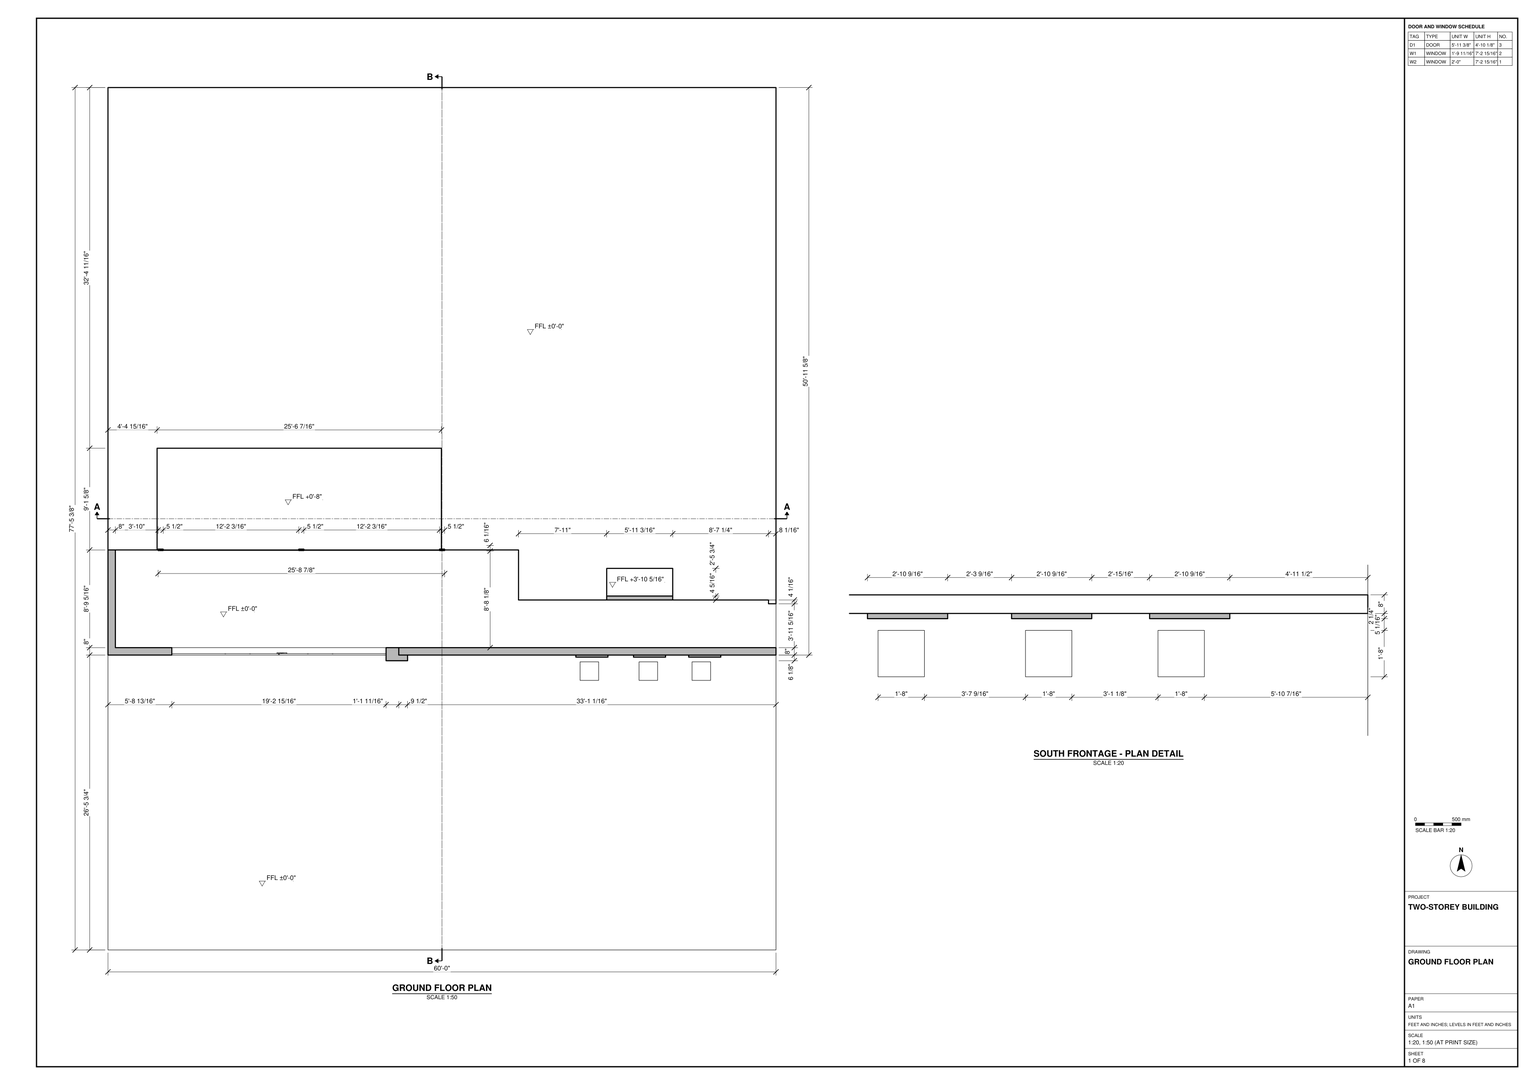
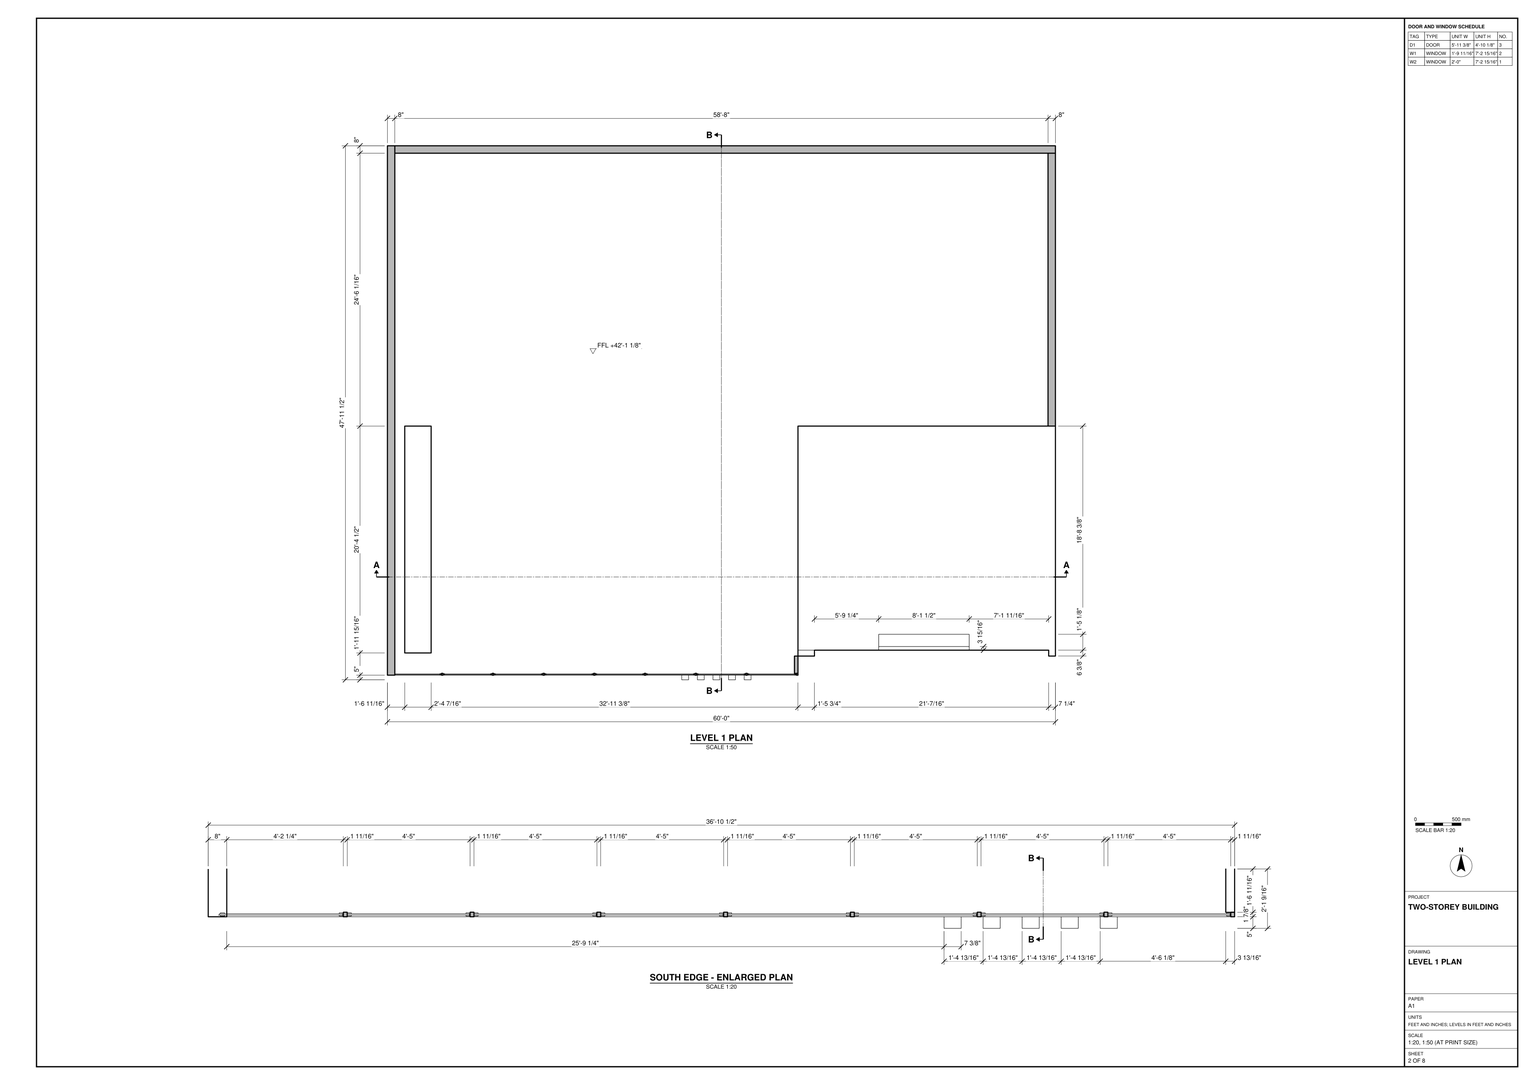
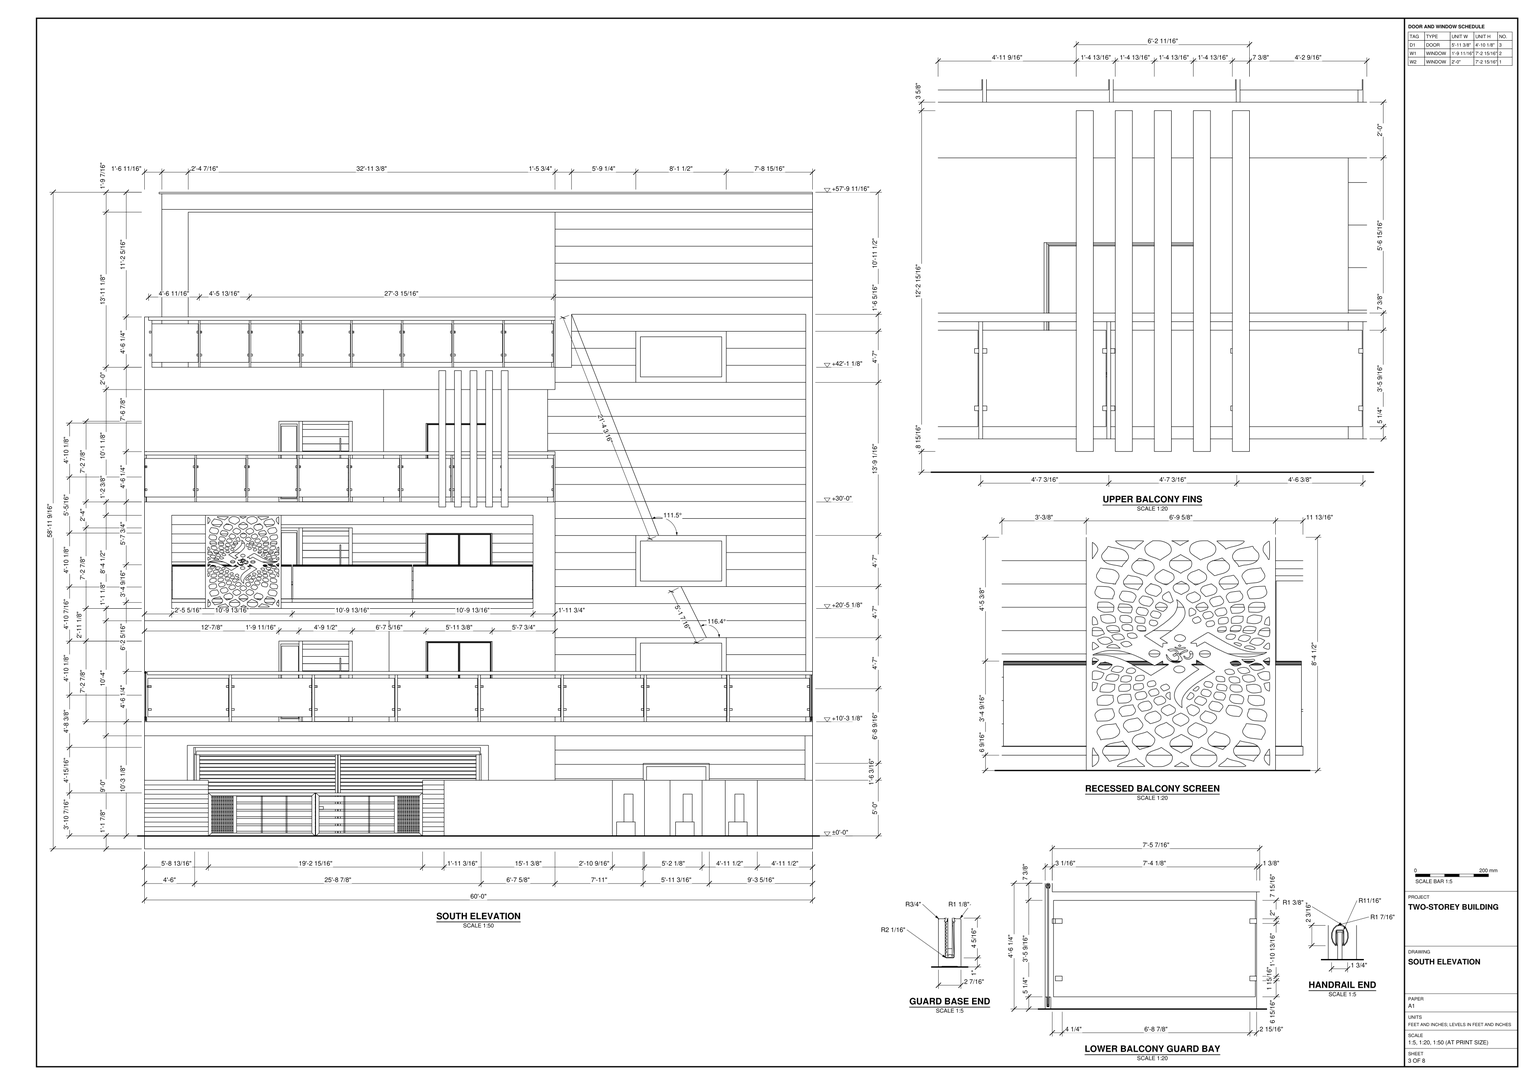
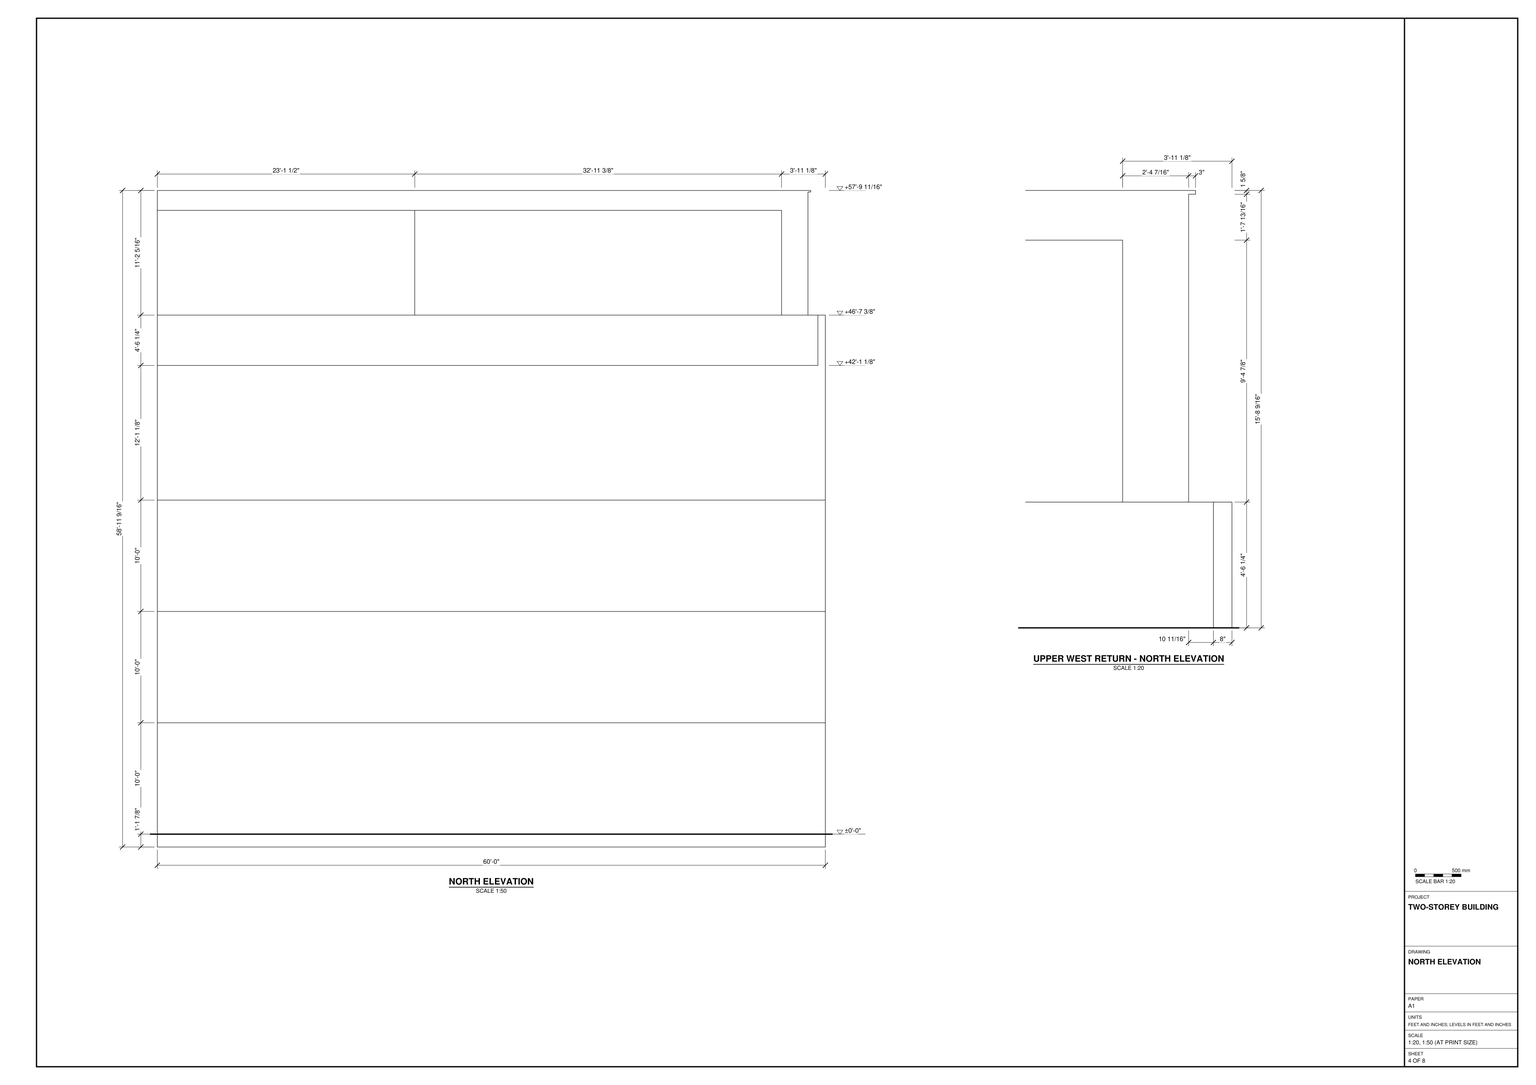
Build the two-storey building in SketchUp from task_files/diagram_01.pdf. Work in feet and inches. The complete model, including the ground area in front of the building, measures 60'-0" along X, 77'-5 3/8" along Y and 58'-11 9/16" in height. Set the ground floor at ±0'-0" and Level 1 at +42'-1 1/8". Use the south elevation to set the intermediate balcony heights rather than spacing the balconies evenly between the storey levels.

Follow the plans for the frontage setback, wall thicknesses, slab outlines and openings. Use the sections to establish slab and roof thicknesses. On the south face, model the wide ground-level gate, the full-width lower balcony and the shorter balconies above it. Include the framed doors and windows behind the guards. Reproduce the horizontal bands and window arrangement on the right-hand wall. Use the enlarged details to place the perforated screen in the recessed balcony and the vertical fins in front of the balcony above. Divide the glass guards into bays with posts and handrails as drawn.

Include stairs, built-in joinery and main furniture only where shown. Keep shell elements such as walls, slabs and roof, and each furniture or joinery piece, in separate groups or components. Use components for repeated parts such as guard bays. Decor and loose items may be any suitable library components. Save one SketchUp model as output_files/two_storey_building_with_stacked_south_facing_balconies.skp.

# SketchUp Ruby script. Lengths in inches.
U = 1.inch
M = Sketchup.active_model
def pt(a) = Geom::Point3d.new(a.map { |v| v * U })
def face(e, loops, mat)
  f = e.add_face(loops[0].map { |a| pt(a) })
  loops[1..].each { |l| e.add_face(l.map { |a| pt(a) }).erase! }
  f.material = f.back_material = mat if mat
  f
end
# faces: each face lists its corners as indices into pts; further lists are holes
def faces(e, pts, list, mat = nil) = list.each { |f| face(e, (f[0].is_a?(Array) ? f : [f]).map { |l| l.map { |i| pts[i] } }, mat) }
# xy, xz, yz: faces in a plane at the given z, y or x. An outline is a flat list of corners, or four numbers for a rectangle; further outlines are holes
def ring(l) = l.size == 4 ? [[l[0], l[1]], [l[2], l[1]], [l[2], l[3]], [l[0], l[3]]] : l.each_slice(2).to_a
def flat(e, list, mat, &to3) = list.each { |f| face(e, (f[0].is_a?(Array) ? f : [f]).map { |l| ring(l).map { |u, v| to3.(u, v) } }, mat) }
def xy(e, z, list, mat = nil) = flat(e, list, mat) { |x, y| [x, y, z] }
def xz(e, y, list, mat = nil) = flat(e, list, mat) { |x, z| [x, y, z] }
def yz(e, x, list, mat = nil) = flat(e, list, mat) { |y, z| [x, y, z] }
def lines(e, pts, list) = list.each { |a, b| e.add_line(pt(pts[a]), pt(pts[b])) }
# prism: a flat outline (further loops are holes) pulled along v
def prism(e, loops, v, mat = nil)
  f = face(e, loops, mat); d = Geom::Vector3d.new(v.map { |x| x * U })
  f.pushpull(f.normal.samedirection?(d) ? d.length : -d.length)
end
def box(e, o, s, mat = nil) = prism(e, [[o, [o[0] + s[0], o[1], o[2]], [o[0] + s[0], o[1] + s[1], o[2]], [o[0], o[1] + s[1], o[2]]]], [0, 0, s[2]], mat)
def at(x, y, z, deg = 0) = Geom::Transformation.translation(pt([x, y, z])) * Geom::Transformation.rotation(ORIGIN, Z_AXIS, deg.degrees)
def axes(o, x, y, z) = Geom::Transformation.new([*x, 0, *y, 0, *z, 0, *pt(o).to_a, 1])
def part(name) = M.definitions.add(name)
# library, detail: a bought-in or finely detailed component or shape, given as its bounding box
def library(name, o, s) = part(name).tap { |d| box(d.entities, o, s) }
def detail(e, o, s) = box(e.add_group.entities, o, s)
def put(e, d, t, mat = nil) = e.add_instance(d, t).tap { |i| i.material = mat if mat }
def group(e, t, mat = nil) = e.add_group.tap { |g| g.transformation = t; g.material = mat if mat }.entities
root = M.entities
M.materials.add("[0029_BlanchedAlmond]").color = [255, 235, 205]
M.materials.add("[0050_LemonChiffon]").color = [255, 250, 205]
M.materials.add("[0131_Silver]").color = [28, 28, 28]
M.materials.add("[0135_DarkGray]1").color = [81, 81, 81]
M.materials.add("[Color_000]").color = [255, 255, 255]
M.materials.add("[Granite Dark Gray]").color = [69, 68, 68]
M.materials.add("[Granite Light Gray]").color = [149, 148, 144]
M.materials.add("[Sandstone]").color = [118, 81, 52]
M.materials.add("[Slate Light Tile]").color = [53, 53, 53]
M.materials.add("[Translucent Glass Blue]").color = [100, 149, 237]
M.materials["[Translucent Glass Blue]"].alpha = 0.5
M.materials.add("[Translucent_Glass_Blue]").color = [255, 255, 255]
M.materials["[Translucent_Glass_Blue]"].alpha = 0
M.materials.add("[Wood Cherry Original]").color = [68, 39, 18]
M.materials.add("[Wood Cherry Original]1").color = [152, 86, 42]
M.materials.add("[Wood Floor Light]").color = [140, 99, 62]
c1 = part("Group\#11")
xy(c1.entities,0,[[0,0,0.39,2.125]],"[0131_Silver]")
xy(c1.entities,1.5,[[0,0,0.39,2.125]],"[0131_Silver]")
xz(c1.entities,0,[[0,0,0.39,1.5]],"[0131_Silver]")
xz(c1.entities,2.125,[[0,0,0.39,1.5]],"[0131_Silver]")
yz(c1.entities,0,[[0,0,2.125,1.5]],"[0131_Silver]")
yz(c1.entities,0.39,[[0,0,2.125,1.5]],"[0131_Silver]")
c2 = part("Glass railing panel")
xy(c2.entities,0,[[-0.59,0,0,63.98]])
xy(c2.entities,37.71,[[-0.59,0,0,63.98]])
xz(c2.entities,0,[[-0.59,0,0,37.71]])
xz(c2.entities,63.98,[[-0.59,0,0,37.71]])
yz(c2.entities,-0.59,[[0,0,63.98,37.71]])
yz(c2.entities,0,[[0,0,63.98,0,63.98,37.71,0,37.71,0,30.53,1.75,30.53,1.75,28.71,0,28.71],[-0.4,28.71,0,30.53],[0,28.71,1.75,30.53]])
p = [[0,63.98,30.53],[0.39,63.98,30.53]]
lines(c2.entities,p,[[0,1]])
put(c2.entities,c1,axes([0,62.22,28.71],[1,0,0],[0,1.01246,0],[0,0,1.2158]))
put(c2.entities,c1,axes([0,62.22,6.27],[1,0,0],[0,1.01246,0],[0,0,1.2158]))
put(c2.entities,c1,axes([0,0.6,28.71],[1,0,0],[0,1.01246,0],[0,0,1.2158]))
put(c2.entities,c1,axes([0,0.6,6.27],[1,0,0],[0,1.01246,0],[0,0,1.2158]))
put(c2.entities,c1,axes([-0.98,0.6,28.71],[1,0,0],[0,1.01246,0],[0,0,1.2158]))
put(c2.entities,c1,axes([-0.98,62.22,6.27],[1,0,0],[0,1.01246,0],[0,0,1.2158]))
put(c2.entities,c1,axes([-0.98,0.6,6.27],[1,0,0],[0,1.01246,0],[0,0,1.2158]))
put(c2.entities,c1,axes([-0.98,62.22,28.71],[1,0,0],[0,1.01246,0],[0,0,1.2158]))
c3 = part("Group\#1")
xz(c3.entities,0,[[0,0,1.97,38.58]])
xz(c3.entities,1.97,[[0,0,1.97,38.58]])
yz(c3.entities,0,[[0,0,1.97,37.71]])
yz(c3.entities,1.97,[[0,0,1.97,37.71]])
c4 = part("Glass railing run")
xy(c4.entities,37.71,[[2.51,0,3.15,0.39,3.15,0]])
xy(c4.entities,37.71,[[0,0,0.54,520.67],[2.51,0,2.51,63.58,3.15,0.39],[3.15,0.39,2.51,63.58,2.51,520.67,3.15,520.67]],"[0131_Silver]")
xy(c4.entities,38.58,[[0.54,496.0625,2.51,520.67]])
xy(c4.entities,38.58,[[0.54,0,2.51,496.0625]],"[0131_Silver]")
xy(c4.entities,40.46,[[0,0,3.15,520.67]],"[0131_Silver]")
xz(c4.entities,0,[[0,37.71,0.54,37.71,0.54,38.58,2.51,38.58,2.51,37.71,3.15,37.71,3.15,40.46,0,40.46]],"[0131_Silver]")
xz(c4.entities,520.67,[[0,37.71,0,40.46,3.15,40.46,3.15,37.71,2.51,37.71,2.51,38.58,0.54,38.58,0.54,37.71]])
yz(c4.entities,0,[[0,37.71,520.67,40.46]],"[0131_Silver]")
yz(c4.entities,0.54,[[496.0625,37.71,520.67,38.58]])
yz(c4.entities,0.54,[[0,37.71,496.0625,38.58]],"[0131_Silver]")
yz(c4.entities,2.51,[[0,37.71,496.0625,38.58],[496.0625,37.71,520.67,38.58]])
yz(c4.entities,3.15,[[0,37.71,520.67,40.46]],"[0131_Silver]")
put(c4.entities,c2,axes([1.8,65.35,3.9375],[1,0,0],[0,0.98769,0],[0,0,0.8225]),"[Translucent_Glass_Blue]")
put(c4.entities,c2,axes([1.8,130.31,3.9375],[1,0,0],[0,0.98769,0],[0,0,0.8225]),"[Translucent_Glass_Blue]")
put(c4.entities,c2,axes([1.8,195.28,3.9375],[1,0,0],[0,0.98769,0],[0,0,0.8225]),"[Translucent_Glass_Blue]")
put(c4.entities,c2,axes([1.8,260.24,3.9375],[1,0,0],[0,0.98769,0],[0,0,0.8225]),"[Translucent_Glass_Blue]")
put(c4.entities,c2,axes([1.8,325.2,3.9375],[1,0,0],[0,0.98769,0],[0,0,0.8225]),"[Translucent_Glass_Blue]")
put(c4.entities,c2,axes([1.8,390.16,3.9375],[1,0,0],[0,0.98769,0],[0,0,0.8225]),"[Translucent_Glass_Blue]")
put(c4.entities,c2,axes([1.8,455.12,3.9375],[1,0,0],[0,0.98769,0],[0,0,0.8225]),"[Translucent_Glass_Blue]")
put(c4.entities,c2,axes([1.8,0.39,3.9375],[1,0,0],[0,0.98769,0],[0,0,0.8225]),"[Translucent_Glass_Blue]")
put(c4.entities,c3,at(0.54,128.9375,0),"[0131_Silver]")
g1 = group(c4.entities,at(0.54,63.98,0),"[0131_Silver]")
xz(g1,0,[[0,0,1.97,38.58]])
xz(g1,1.97,[[0,0,1.97,38.58]])
yz(g1,0,[[0,0,1.97,37.71]])
yz(g1,1.97,[[0,0,1.97,37.71]])
put(c4.entities,c3,at(0.54,193.9,0),"[0131_Silver]")
put(c4.entities,c3,at(0.54,258.86,0),"[0131_Silver]")
put(c4.entities,c3,at(0.54,323.82,0),"[0131_Silver]")
put(c4.entities,c3,at(0.54,388.78,0),"[0131_Silver]")
put(c4.entities,c3,at(0.54,453.74,0),"[0131_Silver]")
put(c4.entities,c3,at(0.54,518.7,0),"[0131_Silver]")
c5 = part("Glass Railing")
put(c5.entities,c4,axes([0,0,0],[1,0,0],[0,0.95652,0],[0,0,1]),"[0131_Silver]")
c6 = library("Glass Railings(black Handrails)",[-57.04,-132.55,0],[169.29,2.52,28.17])
c7 = part("Agrupar\#4")
xy(c7.entities,0,[[0,0,60.82,4.875]],"[Wood Floor Light]")
c8 = part("Agrupar\#7")
box(c8.entities,[0,0,0.25],[0.65,5.875,0.35])
c9 = part("Agrupar\#15")
prism(c9.entities,[[[0,0.625,0],[0.65,0.625,0],[0.65,0,0],[0,0,0]]],[0,0.02,45.16])
c10 = part("Agrupar\#14")
put(c10.entities,c8,at(0,0.65,6.88))
put(c10.entities,c9,at(0,0,0))
put(c10.entities,c8,at(0,0.65,40.25))
c11 = part("Agrupar\#6")
prism(c11.entities,[[[-0.5,0.62,-4.9375],[0.77,0.62,-4.9375],[0.77,-0.19,-4.9375],[-0.5,-0.19,-4.9375]]],[0,0.03,52.91])
c12 = part("Agrupar\#8")
put(c12.entities,c8,at(0,0.65,6.88))
put(c12.entities,c11,at(0,0,0))
put(c12.entities,c8,at(0,0.65,40.25))
c13 = part("Agrupar\#2")
prism(c13.entities,[[[0,2.67,0.04],[55.46,2.67,0.04],[55.46,0.04,0],[0,0.04,0]]],[0,-0.04,3.23],"[Wood Cherry Original]")
c14 = part("Agrupar\#10")
prism(c14.entities,[[[0,3.76,0.04],[4.23,3.76,0.04],[4.23,1.14,0],[0,1.14,0]]],[0,-1.14,83.14],"[Wood Cherry Original]")
c15 = part("Agrupar\#1")
prism(c15.entities,[[[0,3.76,0.04],[4.23,3.76,0.04],[4.23,1.14,0],[0,1.14,0]]],[0,-1.14,83.14],"[Wood Cherry Original]")
c16 = part("Agrupar\#3")
put(c16.entities,c13,at(4.23,0,79.91))
put(c16.entities,c14,at(59.6875,0,0))
put(c16.entities,c15,at(0,0,0))
c17 = part("Agrupar\#5")
put(c17.entities,c16,axes([0,-1.34,0.11],[1,0,0],[0,3.10443,-0.05961],[0,0.0192,0.99982]))
c18 = part("Agrupar\#9")
put(c18.entities,c10,axes([49.36,10.72,17.77],[1,0,0],[0,-1,0],[0,0,1]))
put(c18.entities,c12,at(49.36,0,17.76))
put(c18.entities,c17,at(0,0.21,0.01))
c19 = part("Agrupar\#11")
box(c19.entities,[0,0,0],[60.82,4.875,7.44],"[Wood Floor Light]")
c20 = part("Agrupar\#12")
put(c20.entities,c19,at(0,0,67.34))
put(c20.entities,c19,at(0,0,44.83))
put(c20.entities,c19,at(0,0,59.9))
put(c20.entities,c19,at(0,0,74.78))
put(c20.entities,c19,at(0,0,52.37))
put(c20.entities,c19,at(0,0,7.53))
put(c20.entities,c19,at(0,0,0))
put(c20.entities,c19,at(0,0,29.95))
put(c20.entities,c19,at(0,0,15.07))
put(c20.entities,c19,at(0,0,22.51))
put(c20.entities,c19,at(0,0,37.39))
c21 = part("Agrupar\#13")
put(c21.entities,c18,at(0,0,0.0625))
put(c21.entities,c20,axes([2.375,5.17,0.15],[1,0,0],[0,0.48232,0.01095],[0,-0.02269,0.99974]))
c22 = part("PORTA PIVOTANDE ENVERNIZADA LUXURY")
p = [[59.6875,-1.28,79.91],[59.6875,-3.1,79.89],[4.23,-1.28,79.91],[4.23,-3.1,79.89]]
lines(c22.entities,p,[[0,1],[2,3]])
put(c22.entities,c7,at(0.13,-2.89,82.23))
put(c22.entities,c21,at(0,-6.8,-0.11))
c23 = part("bod vindu")
g2 = group(c23.entities,at(0,-46.85,0),"[Translucent Glass Blue]")
yz(g2,0.94,[[2.36,2.36,44.49,19.65]],"[Translucent Glass Blue]")
p = [[0.55,44.49,2.36],[0.94,44.49,2.36],[0.55,2.36,19.65],[0.94,2.36,19.65]]
lines(g2,p,[[0,1],[2,3]])
g3 = group(g2,at(0,46.85,0,-90),"[Color_000]")
xy(g3,0,[[0,0,46.85,3.9375]])
xy(g3,1.57,[[1.57,0,45.28,0.55]])
xy(g3,2.36,[[2.36,0.55,44.49,3.9375]])
xy(g3,19.65,[[2.36,0.55,4.29,3.9375],[4.29,0.55,44.49,3.9375]])
xy(g3,20.43,[[1.57,0,45.28,0.55]])
xy(g3,22.01,[[0,0,46.85,3.9375]])
xz(g3,0,[[[0,0,46.85,22.01],[1.57,1.57,45.28,20.43]]])
xz(g3,0.55,[[1.57,1.57,45.28,2.36],[1.57,2.36,2.36,2.36,2.36,19.65,44.49,19.65,44.49,2.36,45.28,2.36,45.28,20.43,1.57,20.43]])
xz(g3,3.9375,[[[0,0,46.85,22.01],[2.36,2.36,44.49,19.65]]])
yz(g3,0,[[0,0,3.9375,22.01]])
yz(g3,1.57,[[0,1.57,0.55,2.36,0.55,20.43,0,20.43]])
yz(g3,2.36,[[0.55,2.36,3.9375,19.65]])
yz(g3,44.49,[[0.55,2.36,3.9375,19.65]])
yz(g3,45.28,[[0,1.57,0,20.43,0.55,20.43,0.55,2.36]])
yz(g3,46.85,[[0,0,3.9375,22.01]])
p = [[45.28,0,1.57],[1.57,0,1.57],[1.57,0.55,2.36],[2.36,0.55,2.36],[44.49,0.55,2.36],[45.28,0.55,2.36]]
faces(g3,p,[[0,1,2,3,4,5]])
c24 = library("CNC Jali design 2",[0,0,0],[120,1.08,239.44])
c25 = library("Untitled",[514.11,211.85,0],[136,6,108])
c26 = library("window",[0,0,0],[24,5.5,84.25])
c27 = library("Untitled\#1",[131.66,19.68,0],[2.41,197.25,46.46])
c28 = library("Group\#264",[0,0,0],[99.27,23.72,99.27])
xy(root,-13.875,[[0,0,720,929.375]])
xy(root,0,[[299.74,311.66,302.74,317.78],[302.74,311.66,322.93,317.78],[504.29,315.53,538.86,317.78],[566.42,315.53,600.99,317.78],[625.93,315.53,660.49,317.78],
  [68.8,317.78,299.74,325.78],[299.74,317.78,302.74,325.78],[302.74,317.78,313.43,325.78],[8,325.78,720,325.78,720,377.125,442.51,377.125,442.51,431.0625,8,431.0625],[442.51,377.125,720,377.125,720,929.375,0,929.375,0,431.0625,442.51,431.0625]])
xy(root,0,[[[0,0,720,0,720,317.78,660.49,317.78,660.49,315.53,625.93,315.53,625.93,317.78,600.99,317.78,600.99,315.53,566.42,315.53,566.42,317.78,538.86,317.78,538.86,315.53,504.29,315.53,504.29,317.78,322.93,317.78,322.93,311.66,299.74,311.66,299.74,317.78,0,317.78],[508.85,290.48,528.85,310.48],[572.41,290.48,592.41,310.48],[629.53,290.48,649.53,310.48]]],"[Slate Light Tile]")
xy(root,8.02,[[52.94,431.0625,359.37,540.6875]])
xy(root,12.3,[[516.79,315.53,526.6,316.59],[580.54,315.53,590.35,316.53],[636.29,315.53,646.1,317.34]])
xy(root,15.125,[[508.85,290.48,528.85,310.48],[572.41,290.48,592.41,310.48],[629.53,290.48,649.53,310.48]],"[Wood Cherry Original]1")
xy(root,30.86,[[711.92,373.0625,720,377.125]])
xy(root,45.11,[[516.79,315.53,526.6,316.59],[580.54,315.53,590.35,316.53],[636.29,315.53,646.1,317.34]])
xy(root,46.29,[[537.55,377.125,608.69,411.1875]],"[0029_BlanchedAlmond]")
xy(root,60,[[625.93,315.53,660.49,317.78]])
xy(root,60,[[299.74,311.66,322.93,311.66,322.93,317.78,313.43,317.78,313.43,325.78,299.74,325.78],[0,317.78,68.8,317.78,68.8,325.78,8,325.78,8,431.0625,0,431.0625],[313.43,317.78,720,325.78]],"[0135_DarkGray]1")
xy(root,60,[[504.29,315.53,538.86,317.78],[566.42,315.53,600.99,317.78]],"[Sandstone]")
xy(root,77.14,[[537.55,377.125,608.69,411.1875]],"[0029_BlanchedAlmond]")
xy(root,95.4,[[52.94,431.0625,359.37,540.6875]])
xy(root,108,[[0,338.0625,0,431.0625,442.51,431.0625,442.51,377.125,711.92,377.125,711.92,373.0625,720,373.0625,720,338.0625]],"[Wood Cherry Original]1")
xy(root,120,[[442.51,377.125,442.51,431.0625,0,431.0625,0,929.375,720,929.375,720,377.125]])
xy(root,123.125,[[0,428.75,144.85,431.0625],[224.03,428.75,263.59,431.0625],[144.85,431.0625,224.03,489.5]])
xy(root,123.125,[[0,338.0625,720,338.0625,720,379.47,712.74,379.47,712.74,385.8125,442.51,385.8125,442.51,431.0625,263.59,431.0625,263.59,428.75,224.03,428.75,224.03,431.0625,144.85,431.0625,144.85,428.75,0,428.75]],"[Wood Cherry Original]1")
xy(root,151.79,[[303.36,431.0625,374.73,457.375]])
xy(root,158.74,[[529.55,385.8125,627.05,401.25]])
xy(root,209.6,[[303.36,431.0625,374.73,457.375]])
xy(root,210.0625,[[144.85,428.75,224.03,489.5]])
xy(root,213.76,[[529.55,385.8125,627.05,401.25]])
xy(root,232,[[0,358.875,0,428.75,263.59,428.75,263.59,431.0625,442.51,431.0625,442.51,358.875]],"[Granite Dark Gray]")
xy(root,245.125,[[29.3125,358.875,418.76,360.125],[29.3125,364.1875,418.76,364.1875,418.76,431.0625,224.03,431.0625,224.03,481.125,144.85,481.125,144.85,431.0625,29.3125,431.0625]],"[Granite Dark Gray]")
xy(root,251.6875,[[29.3125,360.125,418.76,364.1875]],"[Granite Dark Gray]")
xy(root,268.35,[[303.36,431.0625,374.73,449.5]],"[0050_LemonChiffon]")
xy(root,268.78,[[529.55,385.8125,627.05,406.625]])
xy(root,323.8,[[529.55,385.8125,627.05,406.625]])
xy(root,326.16,[[303.36,431.0625,374.73,449.5]])
xy(root,332.0625,[[144.85,431.0625,224.03,481.125]],"[Granite Dark Gray]")
xy(root,345.625,[[29.3125,358.875,418.76,431.0625]],"[Granite Dark Gray]")
xy(root,354.5625,[[317.24,353.875,324.61,358.875],[334.07,353.875,341.44,358.875],[350.89,353.875,358.27,358.875],[367.72,353.875,375.1,358.875],[384.55,353.875,391.92,358.875]])
xy(root,360,[[0,358.875,434.51,358.875,434.51,431.0625,257.67,431.0625,257.67,430.25,224.03,430.25,224.03,466.6875,144.85,466.6875,144.85,430.25,0,430.25],[434.51,358.875,442.51,360.85]])
xy(root,386.79,[[303.36,431.0625,374.73,462.75]])
xy(root,414.22,[[434.51,360.85,442.51,385.8125]])
xy(root,444.6,[[303.36,431.0625,374.73,462.75]])
xy(root,446.9375,[[144.85,430.25,224.03,466.6875]])
xy(root,481.125,[[0,358.875,0,430.25,257.67,430.25,257.67,431.0625,434.51,431.0625,434.51,385.8125,442.51,385.8125,442.51,358.875]])
xy(root,488.85,[[529.55,385.8125,627.05,402.9375]])
xy(root,501.5,[[317.24,353.875,324.61,358.875],[334.07,353.875,341.44,358.875],[350.89,353.875,358.27,358.875],[367.72,353.875,375.1,358.875],[384.55,353.875,391.92,358.875]])
xy(root,505.01,[[442.51,379.47,460.28,385.8125]])
xy(root,505.125,[[[8,358.875,442.51,358.875,442.51,360.78,438.69,360.78,438.69,379.47,442.51,379.47,442.51,627.3125,712,627.3125,712,921.375,8,921.375],[18.6875,382.8125,47.125,627.3125]],[712,627.3125,720,921.375],[8,921.375,720,929.375]])
xy(root,543.87,[[529.55,385.8125,627.05,402.9375]])
xy(root,559.35,[[0,358.875,8,929.375],[438.69,360.78,442.51,379.47],[712,627.3125,720,921.375],[8,921.375,720,929.375]])
xy(root,562.21,[[460.28,379.47,712.74,385.8125]])
xy(root,580.55,[[442.51,379.47,720,385.8125]])
xy(root,672.25,[[442.51,385.8125,720,627.3125]])
xy(root,672.25,[[[47.125,382.8125,47.125,627.3125,442.51,627.3125,442.51,385.8125,720,385.8125,720,382.8125],[86.36,426.125,123.61,569.3125],[278.57,426.125,314.01,569.3125],[354.8,426.125,390.17,569.3125],[242.31,426.125,275.93,569.3125],[128.125,426.125,161.6875,569.3125],[318.9,426.125,352.09,569.3125],[167.21,426.125,199.77,569.3125],[209.16,426.125,237.85,569.3125]]],"[Sandstone]")
xy(root,675.25,[[18.6875,382.8125,720,385.8125]],"[0135_DarkGray]1")
xy(root,692.0625,[[15.6875,382.8125,15.6875,627.3125,18.6875,627.3125,18.6875,385.8125,720,385.8125,720,382.8125]])
xy(root,693.6875,[[[15.6875,382.8125,720,627.3125],[86.36,426.125,123.61,569.3125],[278.57,426.125,314.01,569.3125],[354.8,426.125,390.17,569.3125],[242.31,426.125,275.93,569.3125],[128.125,426.125,161.6875,569.3125],[318.9,426.125,352.09,569.3125],[167.21,426.125,199.77,569.3125],[209.16,426.125,237.85,569.3125]]],"[0135_DarkGray]1")
xz(root,0,[[0,-13.875,720,0]])
xz(root,290.48,[[508.85,0,528.85,15.125],[572.41,0,592.41,15.125],[629.53,0,649.53,15.125]],"[Wood Cherry Original]1")
xz(root,310.48,[[508.85,0,528.85,15.125],[572.41,0,592.41,15.125],[629.53,0,649.53,15.125]])
xz(root,311.66,[[299.74,0,322.93,5],[299.74,5,322.93,10],[299.74,10,322.93,15],[299.74,15,322.93,20],[299.74,20,322.93,25],
  [299.74,25,322.93,30],[299.74,30,322.93,35],[299.74,35,322.93,40],[299.74,40,322.93,45],[299.74,45,322.93,50],
  [299.74,50,322.93,55],[299.74,55,322.93,60]],"[0135_DarkGray]1")
xz(root,315.53,[[[504.29,0,538.86,60],[516.79,12.3,526.6,45.11]],[[566.42,0,600.99,60],[580.54,12.3,590.35,45.11]],[[625.93,0,660.49,60],[636.29,12.3,646.1,45.11]]],"[Sandstone]")
xz(root,316.53,[[580.54,12.3,590.35,45.11]])
xz(root,316.59,[[516.79,12.3,526.6,45.11]])
xz(root,317.34,[[636.29,12.3,646.1,45.11]])
xz(root,317.78,[[313.43,0,322.93,60],[322.93,0,504.29,60],[504.29,0,538.86,60],[538.86,0,566.42,60],[566.42,0,600.99,60],
  [600.99,0,625.93,60],[625.93,0,660.49,60],[660.49,0,720,60]])
xz(root,317.78,[[0,0,68.8,5],[0,5,68.8,10],[0,10,68.8,15],[0,15,68.8,20],[0,20,68.8,25],
  [0,25,68.8,30],[0,30,68.8,35],[0,35,68.8,40],[0,40,68.8,45],[0,45,68.8,50],
  [0,50,68.8,55],[0,55,68.8,60]],"[0135_DarkGray]1")
xz(root,325.78,[[8,0,68.8,60],[299.74,0,313.43,60],[313.43,0,720,60]])
xz(root,338.0625,[[0,108,720,123.125]],"[Wood Cherry Original]1")
xz(root,353.875,[[317.24,354.5625,324.61,501.5],[334.07,354.5625,341.44,501.5],[350.89,354.5625,358.27,501.5],[367.72,354.5625,375.1,501.5],[384.55,354.5625,391.92,501.5]])
xz(root,358.875,[[317.24,354.5625,324.61,360],[334.07,354.5625,341.44,360],[350.89,354.5625,358.27,360],[367.72,354.5625,375.1,360],[384.55,354.5625,391.92,360],
  [317.24,360,324.61,481.125],[334.07,360,341.44,481.125],[350.89,360,358.27,481.125],[367.72,360,375.1,481.125],[384.55,360,391.92,481.125],
  [0,481.125,317.24,481.125,317.24,501.5,324.61,501.5,324.61,481.125,334.07,481.125,334.07,501.5,341.44,501.5,341.44,481.125,350.89,481.125,350.89,501.5,358.27,501.5,358.27,481.125,367.72,481.125,367.72,501.5,375.1,501.5,375.1,481.125,384.55,481.125,384.55,501.5,391.92,501.5,391.92,481.125,442.51,481.125,442.51,505.125,8,505.125,8,559.35,0,559.35],[317.24,481.125,324.61,501.5],[334.07,481.125,341.44,501.5],[350.89,481.125,358.27,501.5],[367.72,481.125,375.1,501.5],
  [384.55,481.125,391.92,501.5]])
xz(root,358.875,[[[0,232,442.51,232,442.51,360,391.92,360,391.92,354.5625,384.55,354.5625,384.55,360,375.1,360,375.1,354.5625,367.72,354.5625,367.72,360,358.27,360,358.27,354.5625,350.89,354.5625,350.89,360,341.44,360,341.44,354.5625,334.07,354.5625,334.07,360,324.61,360,324.61,354.5625,317.24,354.5625,317.24,360,0,360],[29.3125,245.125,418.76,345.625]]],"[Granite Dark Gray]")
xz(root,360.125,[[29.3125,245.125,418.76,251.6875]],"[Granite Dark Gray]")
xz(root,360.78,[[438.69,505.125,442.51,559.35]])
xz(root,360.85,[[434.51,360,442.51,414.22]])
xz(root,364.1875,[[29.3125,245.125,418.76,251.6875]],"[Granite Dark Gray]")
xz(root,373.0625,[[711.92,30.86,720,108]])
xz(root,377.125,[[711.92,0,720,15.43],[711.92,15.43,720,30.86]])
xz(root,377.125,[[442.51,0,711.92,15.43],[442.51,15.43,711.92,30.86],[442.51,30.86,711.92,46.29],[442.51,46.29,537.55,61.71],[608.69,46.29,711.92,61.71],
  [442.51,61.71,537.55,77.14],[608.69,61.71,711.92,77.14],[442.51,77.14,711.92,92.57],[442.51,92.57,711.92,108]],"[0029_BlanchedAlmond]")
xz(root,379.47,[[712.74,123.125,720,140.4],[712.74,140.4,720,158.74],[712.74,158.74,720,177.08],[712.74,177.08,720,195.42],[712.74,195.42,720,213.76],
  [712.74,213.76,720,232.1],[712.74,232.1,720,250.44],[712.74,250.44,720,268.78],[712.74,268.78,720,287.12],[712.74,287.12,720,305.46],
  [712.74,305.46,720,323.8],[712.74,323.8,720,342.14],[712.74,342.14,720,360.48],[712.74,360.48,720,378.82],[712.74,378.82,720,397.16],
  [712.74,397.16,720,415.5],[712.74,415.5,720,433.84],[712.74,433.84,720,452.17],[712.74,452.17,720,470.51],[712.74,470.51,720,488.85],
  [712.74,488.85,720,488.85,720,580.55,442.51,580.55,442.51,505.01,460.28,505.01,460.28,562.21,712.74,562.21],[438.69,505.125,442.51,559.35]])
xz(root,382.8125,[[18.6875,505.125,47.125,505.125,47.125,672.25,720,672.25,720,675.25,18.6875,675.25],[15.6875,692.0625,720,693.6875]],"[0135_DarkGray]1")
xz(root,385.8125,[[442.51,580.55,720,598.89],[442.51,598.89,720,617.23],[442.51,617.23,720,635.57],[442.51,635.57,720,653.91],[442.51,653.91,720,672.25]])
xz(root,385.8125,[[442.51,123.125,627.05,140.4],[442.51,140.4,627.05,158.74],[442.51,158.74,529.55,177.08],[442.51,177.08,529.55,195.42],[442.51,195.42,529.55,213.76],
  [442.51,213.76,605.67,213.76,596.55,232.1,442.51,232.1],[442.51,232.1,596.55,232.1,587.42,250.44,442.51,250.44],[442.51,250.44,587.42,250.44,578.3,268.78,442.51,268.78],[442.51,268.78,529.55,287.12],[442.51,287.12,529.55,305.46],
  [442.51,305.46,529.55,323.8],[442.51,323.8,554.12,323.8,546.9,342.14,442.51,342.14],[442.51,342.14,546.9,342.14,539.68,360.48,442.51,360.48],[442.51,360.48,539.68,360.48,532.46,378.82,442.51,378.82],[442.51,378.82,532.46,378.82,525.24,397.16,442.51,397.16],
  [442.51,397.16,525.24,397.16,518.02,415.5,434.51,415.5,434.51,414.22,442.51,414.22],[434.51,415.5,518.02,415.5,510.81,433.84,434.51,433.84],[434.51,433.84,510.81,433.84,503.59,452.17,434.51,452.17],[434.51,452.17,503.59,452.17,496.37,470.51,434.51,470.51],[434.51,470.51,496.37,470.51,489.15,488.85,442.51,488.85,442.51,481.125,434.51,481.125],
  [442.51,488.85,489.15,488.85,481.93,507.19,460.28,507.19,460.28,505.01,442.51,505.01],[460.28,507.19,481.93,507.19,474.71,525.53,460.28,525.53],[460.28,525.53,474.71,525.53,467.5,543.87,460.28,543.87],[460.28,543.87,467.5,543.87,460.28,562.21]],"[0050_LemonChiffon]")
xz(root,385.8125,[[627.05,123.125,712.74,140.4],[627.05,140.4,712.74,158.74],[627.05,158.74,712.74,177.08],[627.05,177.08,712.74,195.42],[627.05,195.42,712.74,213.76],
  [605.67,213.76,712.74,213.76,712.74,232.1,596.55,232.1],[596.55,232.1,712.74,232.1,712.74,250.44,587.42,250.44],[587.42,250.44,712.74,250.44,712.74,268.78,578.3,268.78],[627.05,268.78,712.74,287.12],[627.05,287.12,712.74,305.46],
  [627.05,305.46,712.74,323.8],[554.12,323.8,712.74,323.8,712.74,342.14,546.9,342.14],[546.9,342.14,712.74,342.14,712.74,360.48,539.68,360.48],[539.68,360.48,712.74,360.48,712.74,378.82,532.46,378.82],[532.46,378.82,712.74,378.82,712.74,397.16,525.24,397.16],
  [525.24,397.16,712.74,397.16,712.74,415.5,518.02,415.5],[518.02,415.5,712.74,415.5,712.74,433.84,510.81,433.84],[510.81,433.84,712.74,433.84,712.74,452.17,503.59,452.17],[503.59,452.17,712.74,452.17,712.74,470.51,496.37,470.51],[496.37,470.51,712.74,470.51,712.74,488.85,489.15,488.85],
  [489.15,488.85,529.55,488.85,529.55,507.19,481.93,507.19],[627.05,488.85,712.74,507.19],[481.93,507.19,529.55,507.19,529.55,525.53,474.71,525.53],[627.05,507.19,712.74,525.53],[474.71,525.53,529.55,525.53,529.55,543.87,467.5,543.87],
  [627.05,525.53,712.74,543.87],[467.5,543.87,712.74,543.87,712.74,562.21,460.28,562.21]],"[0135_DarkGray]1")
xz(root,385.8125,[[18.6875,675.25,720,692.0625]],"[Sandstone]")
xz(root,401.25,[[529.55,158.74,627.05,213.76]])
xz(root,402.9375,[[529.55,488.85,627.05,543.87]])
xz(root,406.625,[[529.55,268.78,627.05,323.8]])
xz(root,411.1875,[[537.55,46.29,608.69,77.14]],"[0029_BlanchedAlmond]")
xz(root,426.125,[[86.36,672.25,123.61,693.6875],[128.125,672.25,161.6875,693.6875],[167.21,672.25,199.77,693.6875],[209.16,672.25,237.85,693.6875],[242.31,672.25,275.93,693.6875],
  [278.57,672.25,314.01,693.6875],[318.9,672.25,352.09,693.6875],[354.8,672.25,390.17,693.6875]])
xz(root,428.75,[[0,123.125,144.85,123.125,144.85,210.0625,224.03,210.0625,224.03,123.125,263.59,123.125,263.59,232,0,232]],"[Granite Dark Gray]")
xz(root,430.25,[[0,360,144.85,360,144.85,446.9375,224.03,446.9375,224.03,360,257.67,360,257.67,481.125,0,481.125]],"[Granite Light Gray]")
xz(root,431.0625,[[0,0,8,60],[0,120,442.51,123.125]])
xz(root,431.0625,[[[263.59,123.125,442.51,232],[303.36,151.79,374.73,209.6]],[[257.67,360,434.51,481.125],[303.36,386.79,374.73,444.6]]],"[0029_BlanchedAlmond]")
xz(root,431.0625,[[224.03,245.125,418.76,255.18],[224.03,255.18,418.76,265.23],[224.03,265.23,418.76,265.23,418.76,275.27,374.73,275.27,374.73,268.35,303.36,268.35,303.36,275.27,224.03,275.27],[224.03,275.27,303.36,285.32],[374.73,275.27,418.76,285.32],
  [224.03,285.32,303.36,295.375],[374.73,285.32,418.76,295.375],[224.03,295.375,303.36,305.42],[374.73,295.375,418.76,305.42],[224.03,305.42,303.36,315.48],
  [374.73,305.42,418.76,315.48],[224.03,315.48,303.36,325.52],[374.73,315.48,418.76,325.52],[29.3125,325.52,144.85,325.52,144.85,332.0625,224.03,332.0625,224.03,325.52,303.36,325.52,303.36,326.16,374.73,326.16,374.73,325.52,418.76,325.52,418.76,335.58,29.3125,335.58]],"[0050_LemonChiffon]")
xz(root,431.0625,[[[8,0,442.51,0,442.51,108,0,108,0,60,8,60],[52.94,8.02,359.37,95.4]]],"[0135_DarkGray]1")
xz(root,431.0625,[[29.3125,245.125,144.85,255.18],[29.3125,255.18,144.85,265.23],[29.3125,265.23,144.85,275.27],[29.3125,275.27,144.85,285.32],[29.3125,285.32,144.85,295.375],
  [29.3125,295.375,144.85,305.42],[29.3125,305.42,144.85,315.48],[29.3125,315.48,144.85,325.52],[29.3125,335.58,418.76,345.625]],"[Granite Dark Gray]")
xz(root,449.5,[[303.36,268.35,374.73,326.16]],"[0050_LemonChiffon]")
xz(root,457.375,[[303.36,151.79,374.73,209.6]],"[0050_LemonChiffon]")
xz(root,462.75,[[303.36,386.79,374.73,444.6]])
xz(root,466.6875,[[144.85,360,224.03,446.9375]])
xz(root,481.125,[[144.85,245.125,224.03,332.0625]],"[Granite Dark Gray]")
xz(root,489.5,[[144.85,123.125,224.03,210.0625]])
xz(root,540.6875,[[52.94,8.02,359.37,95.4]])
xz(root,569.3125,[[86.36,672.25,123.61,693.6875],[128.125,672.25,161.6875,693.6875],[167.21,672.25,199.77,693.6875],[209.16,672.25,237.85,693.6875],[242.31,672.25,275.93,693.6875],
  [278.57,672.25,314.01,693.6875],[318.9,672.25,352.09,693.6875],[354.8,672.25,390.17,693.6875]],"[Sandstone]")
xz(root,627.3125,[[18.6875,505.125,18.6875,692.0625,15.6875,692.0625,15.6875,693.6875,720,693.6875,720,672.25,47.125,672.25,47.125,505.125],[442.51,505.125,442.51,672.25,720,672.25,720,559.35,712,559.35,712,505.125],[712,505.125,720,559.35]])
xz(root,921.375,[[8,505.125,712,559.35],[712,505.125,720,559.35]])
xz(root,929.375,[[0,-13.875,720,0],[0,0,720,120],[0,120,720,240],[0,240,720,360],[0,360,0,559.35,8,559.35,8,505.125,720,505.125,720,360],
  [8,505.125,720,559.35]])
yz(root,0,[[431.0625,120,431.0625,123.125,428.75,123.125,428.75,232,358.875,232,358.875,240,929.375,240,929.375,120],[430.25,240,929.375,360],[430.25,360,430.25,481.125,358.875,481.125,358.875,559.35,929.375,559.35,929.375,360]])
yz(root,0,[[0,-13.875,0,0,317.78,0,317.78,60,431.0625,60,431.0625,0,929.375,0,929.375,-13.875]],"[0135_DarkGray]1")
yz(root,0,[[358.875,240,430.25,360]],"[Granite Dark Gray]")
yz(root,0,[[431.0625,0,431.0625,108,338.0625,108,338.0625,123.125,431.0625,123.125,431.0625,120,929.375,120,929.375,0]],"[Wood Cherry Original]1")
yz(root,8,[[358.875,505.125,921.375,559.35],[921.375,505.125,929.375,559.35]])
yz(root,8,[[325.78,0,431.0625,60]],"[0135_DarkGray]1")
yz(root,15.6875,[[382.8125,692.0625,627.3125,693.6875]])
yz(root,18.6875,[[382.8125,505.125,382.8125,675.25,385.8125,675.25,385.8125,692.0625,627.3125,692.0625,627.3125,505.125]])
yz(root,29.3125,[[358.875,245.125,360.125,245.125,360.125,251.6875,364.1875,251.6875,364.1875,245.125,431.0625,245.125,431.0625,345.625,358.875,345.625]],"[Granite Dark Gray]")
yz(root,47.125,[[382.8125,505.125,627.3125,672.25]])
yz(root,52.94,[[431.0625,8.02,540.6875,95.4]])
yz(root,68.8,[[317.78,0,325.78,60]],"[0135_DarkGray]1")
yz(root,86.36,[[426.125,672.25,569.3125,693.6875]],"[Sandstone]")
yz(root,123.61,[[426.125,672.25,569.3125,693.6875]],"[Sandstone]")
yz(root,128.125,[[426.125,672.25,569.3125,693.6875]],"[Sandstone]")
yz(root,144.85,[[428.75,123.125,489.5,210.0625],[430.25,360,466.6875,446.9375]])
yz(root,144.85,[[431.0625,245.125,481.125,332.0625]],"[Granite Dark Gray]")
yz(root,161.6875,[[426.125,672.25,569.3125,693.6875]],"[Sandstone]")
yz(root,167.21,[[426.125,672.25,569.3125,693.6875]],"[Sandstone]")
yz(root,199.77,[[426.125,672.25,569.3125,693.6875]],"[Sandstone]")
yz(root,209.16,[[426.125,672.25,569.3125,693.6875]],"[Sandstone]")
yz(root,224.03,[[428.75,123.125,489.5,210.0625],[430.25,360,466.6875,446.9375]])
yz(root,224.03,[[431.0625,245.125,481.125,332.0625]],"[Granite Dark Gray]")
yz(root,237.85,[[426.125,672.25,569.3125,693.6875]],"[Sandstone]")
yz(root,242.31,[[426.125,672.25,569.3125,693.6875]],"[Sandstone]")
yz(root,257.67,[[430.25,360,431.0625,481.125]])
yz(root,263.59,[[428.75,123.125,431.0625,232]],"[Granite Dark Gray]")
yz(root,275.93,[[426.125,672.25,569.3125,693.6875]],"[Sandstone]")
yz(root,278.57,[[426.125,672.25,569.3125,693.6875]],"[Sandstone]")
yz(root,299.74,[[311.66,0,325.78,60]],"[0135_DarkGray]1")
yz(root,303.36,[[431.0625,151.79,457.375,209.6],[431.0625,386.79,462.75,444.6]])
yz(root,303.36,[[431.0625,268.35,449.5,326.16]],"[0050_LemonChiffon]")
yz(root,313.43,[[317.78,0,325.78,60]])
yz(root,314.01,[[426.125,672.25,569.3125,693.6875]],"[Sandstone]")
yz(root,317.24,[[353.875,354.5625,358.875,501.5]])
yz(root,318.9,[[426.125,672.25,569.3125,693.6875]],"[Sandstone]")
yz(root,322.93,[[311.66,0,317.78,60]],"[0135_DarkGray]1")
yz(root,324.61,[[353.875,354.5625,358.875,501.5]])
yz(root,334.07,[[353.875,354.5625,358.875,501.5]])
yz(root,341.44,[[353.875,354.5625,358.875,501.5]])
yz(root,350.89,[[353.875,354.5625,358.875,501.5]])
yz(root,352.09,[[426.125,672.25,569.3125,693.6875]],"[Sandstone]")
yz(root,354.8,[[426.125,672.25,569.3125,693.6875]],"[Sandstone]")
yz(root,358.27,[[353.875,354.5625,358.875,501.5]])
yz(root,359.37,[[431.0625,8.02,540.6875,95.4]],"[0029_BlanchedAlmond]")
yz(root,367.72,[[353.875,354.5625,358.875,501.5]])
yz(root,374.73,[[431.0625,151.79,457.375,209.6],[431.0625,386.79,462.75,444.6]])
yz(root,374.73,[[431.0625,268.35,449.5,326.16]],"[0050_LemonChiffon]")
yz(root,375.1,[[353.875,354.5625,358.875,501.5]])
yz(root,384.55,[[353.875,354.5625,358.875,501.5]])
yz(root,390.17,[[426.125,672.25,569.3125,693.6875]],"[Sandstone]")
yz(root,391.92,[[353.875,354.5625,358.875,501.5]])
yz(root,418.76,[[358.875,245.125,358.875,345.625,431.0625,345.625,431.0625,245.125,364.1875,245.125,364.1875,251.6875,360.125,251.6875,360.125,245.125]],"[Granite Dark Gray]")
yz(root,434.51,[[360.85,360,360.85,414.22,385.8125,414.22,385.8125,481.125,431.0625,481.125,431.0625,360]])
yz(root,438.69,[[360.78,505.125,379.47,559.35]])
yz(root,442.51,[[385.8125,123.125,431.0625,232],[358.875,232,385.8125,232,385.8125,414.22,360.85,414.22,360.85,360,358.875,360],[358.875,481.125,385.8125,481.125,385.8125,505.01,379.47,505.01,379.47,559.35,360.78,559.35,360.78,505.125,358.875,505.125],[379.47,505.01,385.8125,505.125],[379.47,505.125,379.47,580.55,385.8125,580.55,385.8125,672.25,627.3125,672.25,627.3125,505.125]])
yz(root,442.51,[[377.125,0,431.0625,108]],"[0029_BlanchedAlmond]")
yz(root,460.28,[[379.47,505.01,385.8125,562.21]])
yz(root,504.29,[[315.53,0,317.78,60]],"[Sandstone]")
yz(root,508.85,[[290.48,0,310.48,15.125]],"[Wood Cherry Original]1")
yz(root,516.79,[[315.53,12.3,316.59,45.11]])
yz(root,526.6,[[315.53,12.3,316.59,45.11]])
yz(root,528.85,[[290.48,0,310.48,15.125]],"[Wood Cherry Original]1")
yz(root,529.55,[[385.8125,158.74,401.25,213.76],[385.8125,268.78,406.625,323.8],[385.8125,488.85,402.9375,543.87]])
yz(root,537.55,[[377.125,46.29,411.1875,61.71],[377.125,61.71,411.1875,77.14]],"[0029_BlanchedAlmond]")
yz(root,538.86,[[315.53,0,317.78,60]],"[Sandstone]")
yz(root,566.42,[[315.53,0,317.78,60]],"[Sandstone]")
yz(root,572.41,[[290.48,0,310.48,15.125]],"[Wood Cherry Original]1")
yz(root,580.54,[[315.53,12.3,316.53,45.11]])
yz(root,590.35,[[315.53,12.3,316.53,45.11]])
yz(root,592.41,[[290.48,0,310.48,15.125]],"[Wood Cherry Original]1")
yz(root,600.99,[[315.53,0,317.78,60]],"[Sandstone]")
yz(root,608.69,[[377.125,46.29,411.1875,61.71],[377.125,61.71,411.1875,77.14]],"[0029_BlanchedAlmond]")
yz(root,625.93,[[315.53,0,317.78,60]],"[Sandstone]")
yz(root,627.05,[[385.8125,158.74,401.25,213.76],[385.8125,268.78,406.625,323.8],[385.8125,488.85,402.9375,543.87]])
yz(root,629.53,[[290.48,0,310.48,15.125]],"[Wood Cherry Original]1")
yz(root,636.29,[[315.53,12.3,317.34,45.11]])
yz(root,646.1,[[315.53,12.3,317.34,45.11]])
yz(root,649.53,[[290.48,0,310.48,15.125]],"[Wood Cherry Original]1")
yz(root,660.49,[[315.53,0,317.78,60]],"[Sandstone]")
yz(root,711.92,[[373.0625,30.86,377.125,108]])
yz(root,712,[[627.3125,505.125,921.375,559.35]])
yz(root,712.74,[[379.47,123.125,385.8125,562.21]])
yz(root,720,[[0,-13.875,929.375,-13.875,929.375,0,325.78,0,325.78,60,317.78,60,317.78,0,0,0],[377.125,120,929.375,120,929.375,240,379.47,240,379.47,123.125,377.125,123.125],[379.47,240,929.375,360],[379.47,360,929.375,360,929.375,505.125,627.3125,505.125,627.3125,672.25,385.8125,672.25,385.8125,580.55,379.47,580.55],[627.3125,505.125,921.375,559.35],
  [921.375,505.125,929.375,559.35],[382.8125,672.25,627.3125,672.25,627.3125,693.6875,382.8125,693.6875,382.8125,692.0625,385.8125,692.0625,385.8125,675.25,382.8125,675.25]])
yz(root,720,[[377.125,0,929.375,0,929.375,120,377.125,120,377.125,123.125,338.0625,123.125,338.0625,108,373.0625,108,373.0625,30.86,377.125,30.86]],"[Wood Cherry Original]1")
p = [[442.51,385.8125,360],[434.51,385.8125,360],[442.51,385.8125,122.0625],[720,385.8125,122.0625],[302.74,317.78,0],[302.74,317.78,60]]
lines(root,p,[[0,1],[2,3],[4,5]])
put(root,c5,axes([3.05,341.73,123.125],[0,-1,0],[1.43957,0,0],[0,0,1.34]))
put(root,c6,axes([160.54,496.74,251.6875],[2.30044,0,0],[0,1,0],[0,0,1.44]))
put(root,c22,axes([166.51,438.99,123.28],[0.9,0,0],[0,1,0],[0,0,1.0426]))
put(root,c23,axes([627.05,389.75,158.74],[0,-1,0],[2.08116,0,0],[0,0,2.49996]))
put(root,c24,axes([65.69,362.12,245.125],[0.68,0,0],[0,-2.9971,0],[0,0,0.41972]))
put(root,c25,axes([-1181.03,215.93,-10.35],[2.38693,0,0],[0,1.01,0],[0,0,1]),"[0029_BlanchedAlmond]")
put(root,c22,axes([166.51,438.99,245.28],[0.9,0,0],[0,1,0],[0,0,1.0426]))
put(root,c22,axes([166.51,438.99,360.15],[0.9,0,0],[0,1,0],[0,0,1.0426]))
put(root,c26,axes([144.85,434.61,123.125],[1,0,0],[0,1,0],[0,0,1.03188]))
put(root,c26,axes([144.85,434.6,245.29],[0.90274,0,0],[0,1.18,0],[0,0,1.03188]))
put(root,c26,axes([144.85,434.6,360.16],[0.90274,0,0],[0,1.18,0],[0,0,1.03188]))
put(root,c5,axes([0,361.38,360],[0,-1,0],[0.88851,0,0],[0,0,1.34]))
put(root,c6,axes([845.79,354.92,123.125],[0,0.27521,0],[0.96736,0,0],[0,0,1.9281]))
put(root,c6,axes([128.22,369.28,123.125],[0,0.55042,0],[0.96736,0,0],[0,0,1.9281]))
put(root,c6,axes([28.52,383.95,360.3],[0,0.41968,0],[0.20293,0,0],[0,0,1.9281]))
put(root,c23,axes([627.05,389.75,268.78],[0,-1,0],[2.08116,0,0],[0,0,2.49996]))
put(root,c23,axes([627.05,389.75,488.85],[0,-1,0],[2.08116,0,0],[0,0,2.49996]))
put(root,c5,axes([4.43,361.38,505.125],[0,-1,0],[0.87963,0,0],[0,0,1.34]))
put(root,c23,axes([608.69,381.41,46.29],[0,-1.0885,0],[1.51925,0,0],[0,0,1.44998]))
put(root,c27,axes([45.75,451.85,0],[0,-1,0],[1.17083,0,0],[0,0,1]))
put(root,c28,axes([303.36,431.0625,151.79],[0.71898,0,0],[0,0.86553,0],[0,0,0.58552]))
put(root,c28,axes([303.36,431.0625,268.35],[0.71898,0,0],[0,0.86553,0],[0,0,0.58552]))
put(root,c28,axes([303.36,431.0625,386.79],[0.71898,0,0],[0,0.86553,0],[0,0,0.58552]))
